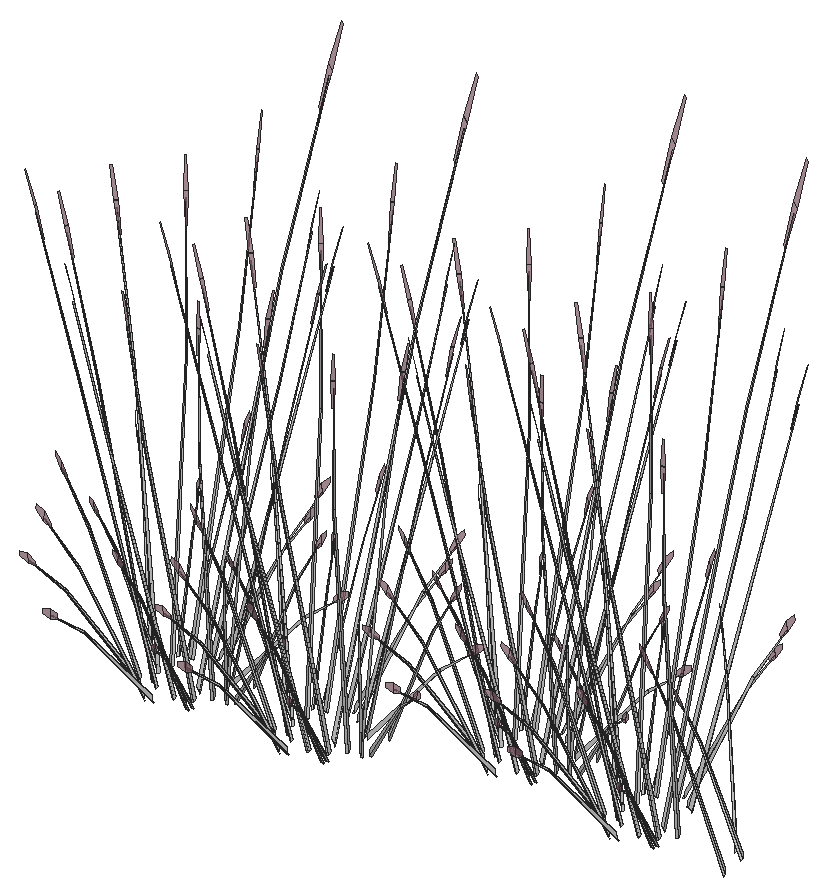
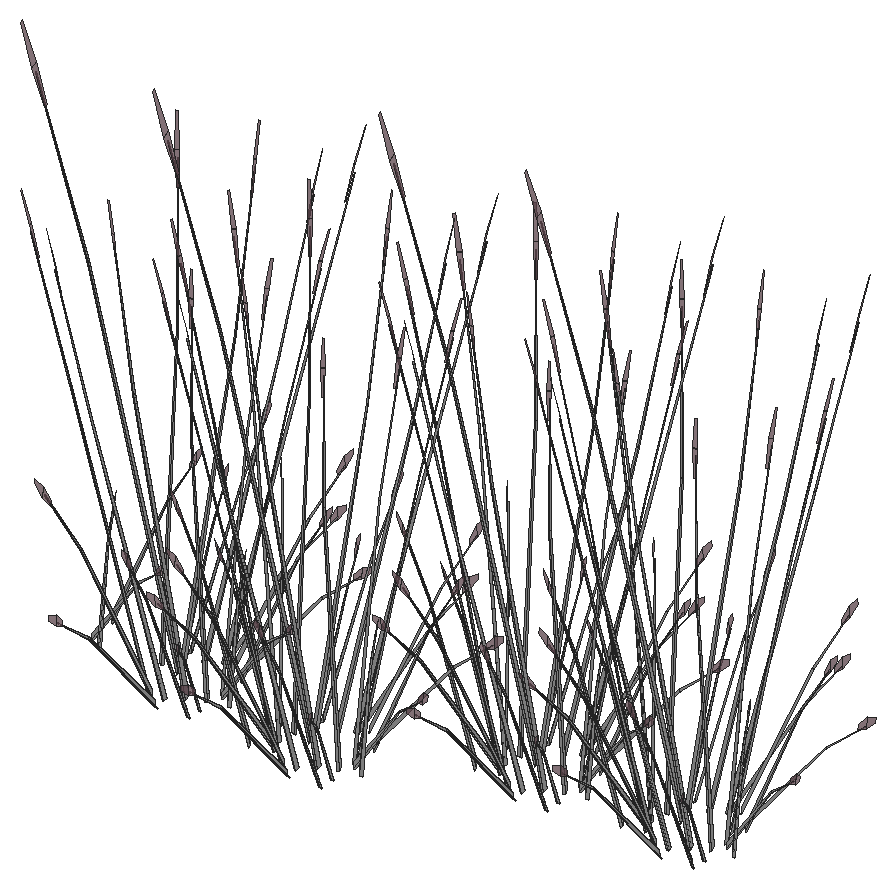
# SketchUp Ruby script. Lengths in inches.
U = 1.inch
M = Sketchup.active_model
def pt(a) = Geom::Point3d.new(a.map { |v| v * U })
def face(e, loops, mat)
  f = e.add_face(loops[0].map { |a| pt(a) })
  loops[1..].each { |l| e.add_face(l.map { |a| pt(a) }).erase! }
  f.material = f.back_material = mat if mat
  f
end
# faces: each face lists its corners as indices into pts; further lists are holes
def faces(e, pts, list, mat = nil) = list.each { |f| face(e, (f[0].is_a?(Array) ? f : [f]).map { |l| l.map { |i| pts[i] } }, mat) }
# xy, xz, yz: faces in a plane at the given z, y or x. An outline is a flat list of corners, or four numbers for a rectangle; further outlines are holes
def ring(l) = l.size == 4 ? [[l[0], l[1]], [l[2], l[1]], [l[2], l[3]], [l[0], l[3]]] : l.each_slice(2).to_a
def flat(e, list, mat, &to3) = list.each { |f| face(e, (f[0].is_a?(Array) ? f : [f]).map { |l| ring(l).map { |u, v| to3.(u, v) } }, mat) }
def xy(e, z, list, mat = nil) = flat(e, list, mat) { |x, y| [x, y, z] }
def xz(e, y, list, mat = nil) = flat(e, list, mat) { |x, z| [x, y, z] }
def yz(e, x, list, mat = nil) = flat(e, list, mat) { |y, z| [x, y, z] }
def lines(e, pts, list) = list.each { |a, b| e.add_line(pt(pts[a]), pt(pts[b])) }
# prism: a flat outline (further loops are holes) pulled along v
def prism(e, loops, v, mat = nil)
  f = face(e, loops, mat); d = Geom::Vector3d.new(v.map { |x| x * U })
  f.pushpull(f.normal.samedirection?(d) ? d.length : -d.length)
end
def box(e, o, s, mat = nil) = prism(e, [[o, [o[0] + s[0], o[1], o[2]], [o[0] + s[0], o[1] + s[1], o[2]], [o[0], o[1] + s[1], o[2]]]], [0, 0, s[2]], mat)
def at(x, y, z, deg = 0) = Geom::Transformation.translation(pt([x, y, z])) * Geom::Transformation.rotation(ORIGIN, Z_AXIS, deg.degrees)
def axes(o, x, y, z) = Geom::Transformation.new([*x, 0, *y, 0, *z, 0, *pt(o).to_a, 1])
def part(name) = M.definitions.add(name)
# library, detail: a bought-in or finely detailed component or shape, given as its bounding box
def library(name, o, s) = part(name).tap { |d| box(d.entities, o, s) }
def detail(e, o, s) = box(e.add_group.entities, o, s)
def put(e, d, t, mat = nil) = e.add_instance(d, t).tap { |i| i.material = mat if mat }
def group(e, t, mat = nil) = e.add_group.tap { |g| g.transformation = t; g.material = mat if mat }.entities
root = M.entities
M.materials.add("LightPink_Translucent").color = [144, 107, 117]
M.materials["LightPink_Translucent"].alpha = 0.75
M.materials.add("[_0053_Ivory_]").color = [200, 200, 200]
c1 = part("blade")
p = [[2.15,0.21,22],[0,0.17,0],[0.09,0.45,0],[2.18,0.31,22],[2.29,0.31,22],[0.38,0.45,0],
  [2.48,0.24,33],[2.49,0.24,33],[2.48,0.22,33]]
faces(c1.entities,p,[[0,1,2,3],[4,5,2,3],[6,3,4,7],[8,0,3,6]])
c2 = part("seeds")
p = [[0.3,-0.1,1.38],[-0.01,-0.03,1.59],[-0.01,-0.03,0.03],[0.14,-0.07,-0.07],[0.29,-0.03,3],[0.15,0.01,3.11]]
faces(c2.entities,p,[[0,1,2,3],[1,0,4,5]],"LightPink_Translucent")
c3 = part("blade with seeds")
put(c3.entities,c1,at(0,0,0))
put(c3.entities,c2,axes([2.4,0.25,30.99],[1.5799,-0.05474,1.17369],[-0.12525,1.92788,0.29478],[-0.07173,-0.02425,1.56792]))
put(root,c3,axes([417.2,98.36,131.37],[-0.09918,0.08165,1.74944],[0.00844,0.59653,-0.27667],[-0.22734,0.07758,0.14031]),"[_0053_Ivory_]")
put(root,c3,axes([416.1,98.96,131.36],[0.07751,0.01687,1.77383],[0.23978,0.55562,-0.16761],[-0.15867,0.14583,0.31391]),"[_0053_Ivory_]")
put(root,c3,axes([417.67,95.875,131.36],[0.04503,0.06276,1.77383],[-0.21706,0.56413,-0.16761],[-0.21983,0.00408,0.31391]),"[_0053_Ivory_]")
put(root,c3,axes([418.17,95.5,131.37],[-0.13068,-0.00444,1.74944],[-0.41604,0.44388,-0.27667],[-0.22198,-0.0907,0.14031]),"[_0053_Ivory_]")
put(root,c3,axes([417.84,97.79,131.6875],[0.30559,0.56943,-0.1216],[-0.54237,0.27983,-0.67495],[-0.22856,0.07513,1.02557]),"[_0053_Ivory_]")
put(root,c3,axes([418.52,96.61,131.6875],[-0.03252,0.63953,-0.1216],[-0.61574,-0.01748,-0.67495],[-0.23714,-0.04442,1.02557]),"[_0053_Ivory_]")
put(root,c3,axes([417.22,100.58,131.37],[-0.0151,0.12444,1.74944],[0.42844,0.43292,-0.27667],[-0.11216,0.20472,0.14031]),"[_0053_Ivory_]")
put(root,c3,axes([419.73,95.67,132.08],[-0.40534,0.60286,-0.13619],[-0.58702,-0.34732,-0.75594],[-0.20405,-0.17032,1.14864]),"[_0053_Ivory_]")
put(root,c3,axes([417.86,99.14,131.6875],[0.56181,0.34675,-0.1216],[-0.32367,0.50216,-0.67495],[-0.15873,0.17455,1.02557]),"[_0053_Ivory_]")
put(root,c3,axes([419.57,94.24,131.36],[-0.01133,0.07538,1.77383],[-0.55883,0.27355,-0.16761],[-0.16445,-0.13983,0.31391]),"[_0053_Ivory_]")
put(root,c3,axes([417.17,101.86,131.36],[0.0689,-0.03797,1.77383],[0.5695,0.25254,-0.16761],[-0.01338,0.21027,0.31391]),"[_0053_Ivory_]")
put(root,c3,axes([420.21,94.53,131.37],[-0.0929,-0.08817,1.74944],[-0.61994,0.0559,-0.27667],[-0.09894,-0.21089,0.14031]),"[_0053_Ivory_]")
put(root,c3,axes([418.59,100.3,132.05],[0.6675,0.03116,-0.13498],[-0.01824,0.58993,-0.74919],[-0.04637,0.2272,1.13838]),"[_0053_Ivory_]")
put(root,c3,axes([421.15,95.89,131.6875],[-0.59433,0.29278,-0.1216],[-0.29207,-0.51964,-0.67495],[-0.07842,-0.21898,1.02557]),"[_0053_Ivory_]")
put(root,c3,axes([419.68,102.125,131.37],[0.07699,0.10127,1.74944],[0.6213,0.03978,-0.27667],[0.06248,0.22333,0.14031]),"[_0053_Ivory_]")
put(root,c3,axes([419.82,100.96,131.6875],[0.59433,-0.29278,-0.1216],[0.29207,0.51964,-0.67495],[0.07842,0.21898,1.02557]),"[_0053_Ivory_]")
put(root,c3,axes([422.86,95.16,131.36],[-0.06168,0.04803,1.77383],[-0.60432,-0.16205,-0.16761],[-0.02188,-0.20961,0.31391]),"[_0053_Ivory_]")
put(root,c3,axes([422.38,96.55,131.6875],[-0.6675,-0.03116,-0.1216],[0.01824,-0.58993,-0.67495],[0.04637,-0.2272,1.02557]),"[_0053_Ivory_]")
put(root,c3,axes([421.64,97.76,131.13],[-0.52482,-0.32674,1.38283],[0.55416,-0.50872,0.59665],[0.16933,0.30658,1.33663]),"[_0053_Ivory_]")
put(root,c3,axes([420.76,101.39,131.36],[0.0018,-0.07613,1.77383],[0.52048,-0.3359,-0.16761],[0.18079,0.11989,0.31391]),"[_0053_Ivory_]")
put(root,c3,axes([422.99,95.61,131.37],[-0.00586,-0.12516,1.74944],[-0.49517,-0.36172,-0.27667],[0.07656,-0.21927,0.14031]),"[_0053_Ivory_]")
put(root,c3,axes([429.41,98.36,131.37],[-0.09918,0.08165,1.74944],[0.00844,0.59653,-0.27667],[-0.22734,0.07758,0.14031]),"[_0053_Ivory_]")
put(root,c3,axes([421.23,100.9375,131.6875],[0.36191,-0.53827,-0.1216],[0.52412,0.3101,-0.67495],[0.18219,0.15207,1.02557]),"[_0053_Ivory_]")
put(root,c3,axes([423.11,97.71,131.6875],[-0.56181,-0.34675,-0.1216],[0.32367,-0.50216,-0.67495],[0.15873,-0.17455,1.02557]),"[_0053_Ivory_]")
put(root,c3,axes([428.3125,98.96,131.36],[0.07751,0.01687,1.77383],[0.23978,0.55562,-0.16761],[-0.15867,0.14583,0.31391]),"[_0053_Ivory_]")
put(root,c3,axes([429.88,95.875,131.36],[0.04503,0.06276,1.77383],[-0.21706,0.56413,-0.16761],[-0.21983,0.00408,0.31391]),"[_0053_Ivory_]")
put(root,c3,axes([430.39,95.5,131.37],[-0.13068,-0.00444,1.74944],[-0.41604,0.44388,-0.27667],[-0.22198,-0.0907,0.14031]),"[_0053_Ivory_]")
put(root,c3,axes([430.05,97.79,131.6875],[0.30559,0.56943,-0.1216],[-0.54237,0.27983,-0.67495],[-0.22856,0.07513,1.02557]),"[_0053_Ivory_]")
put(root,c3,axes([430.74,96.61,131.6875],[-0.03252,0.63953,-0.1216],[-0.61574,-0.01748,-0.67495],[-0.23714,-0.04442,1.02557]),"[_0053_Ivory_]")
put(root,c3,axes([424.49,97.56,131.36],[-0.07933,-0.00478,1.77383],[-0.32942,-0.51175,-0.16761],[0.13229,-0.16826,0.31391]),"[_0053_Ivory_]")
put(root,c3,axes([422.45,100.24,131.6875],[0.03252,-0.63953,-0.1216],[0.61574,0.01748,-0.67495],[0.23714,0.04442,1.02557]),"[_0053_Ivory_]")
put(root,c3,axes([423.13,99.0625,131.6875],[-0.30559,-0.56943,-0.1216],[0.54237,-0.27983,-0.67495],[0.22856,-0.07513,1.02557]),"[_0053_Ivory_]")
put(root,c3,axes([422.98,99.86,131.37],[0.13029,-0.01064,1.74944],[0.35737,-0.48855,-0.27667],[0.23175,0.06449,0.14031]),"[_0053_Ivory_]")
put(root,c3,axes([429.43,100.58,131.37],[-0.0151,0.12444,1.74944],[0.42844,0.43292,-0.27667],[-0.11216,0.20472,0.14031]),"[_0053_Ivory_]")
put(root,c3,axes([431.94,95.67,132.08],[-0.40534,0.60286,-0.13619],[-0.58702,-0.34732,-0.75594],[-0.20405,-0.17032,1.14864]),"[_0053_Ivory_]")
put(root,c3,axes([430.07,99.14,131.6875],[0.56181,0.34675,-0.1216],[-0.32367,0.50216,-0.67495],[-0.15873,0.17455,1.02557]),"[_0053_Ivory_]")
put(root,c3,axes([424.35,100.75,131.36],[-0.05492,-0.05505,1.77383],[0.12013,-0.59013,-0.16761],[0.21632,-0.0377,0.31391]),"[_0053_Ivory_]")
put(root,c3,axes([431.78,94.24,131.36],[-0.01133,0.07538,1.77383],[-0.55883,0.27355,-0.16761],[-0.16445,-0.13983,0.31391]),"[_0053_Ivory_]")
put(root,c3,axes([424.79,98.17,131.37],[0.08428,-0.09579,1.74944],[-0.10787,-0.58756,-0.27667],[0.21147,-0.1114,0.14031]),"[_0053_Ivory_]")
put(root,c3,axes([429.38,101.86,131.36],[0.0689,-0.03797,1.77383],[0.5695,0.25254,-0.16761],[-0.01338,0.21027,0.31391]),"[_0053_Ivory_]")
put(root,c3,axes([432.42,94.53,131.37],[-0.0929,-0.08817,1.74944],[-0.61994,0.0559,-0.27667],[-0.09894,-0.21089,0.14031]),"[_0053_Ivory_]")
put(root,c3,axes([430.8,100.3,132.05],[0.6675,0.03116,-0.13498],[-0.01824,0.58993,-0.74919],[-0.04637,0.2272,1.13838]),"[_0053_Ivory_]")
put(root,c3,axes([433.36,95.89,131.6875],[-0.59433,0.29278,-0.1216],[-0.29207,-0.51964,-0.67495],[-0.07842,-0.21898,1.02557]),"[_0053_Ivory_]")
put(root,c3,axes([431.9,102.125,131.37],[0.07699,0.10127,1.74944],[0.6213,0.03978,-0.27667],[0.06248,0.22333,0.14031]),"[_0053_Ivory_]")
put(root,c3,axes([432.04,100.96,131.6875],[0.59433,-0.29278,-0.1216],[0.29207,0.51964,-0.67495],[0.07842,0.21898,1.02557]),"[_0053_Ivory_]")
put(root,c3,axes([435.07,95.16,131.36],[-0.06168,0.04803,1.77383],[-0.60432,-0.16205,-0.16761],[-0.02188,-0.20961,0.31391]),"[_0053_Ivory_]")
put(root,c3,axes([434.6,96.55,131.6875],[-0.6675,-0.03116,-0.1216],[0.01824,-0.58993,-0.67495],[0.04637,-0.2272,1.02557]),"[_0053_Ivory_]")
put(root,c3,axes([433.86,97.76,131.13],[-0.52482,-0.32674,1.38283],[0.55416,-0.50872,0.59665],[0.16933,0.30658,1.33663]),"[_0053_Ivory_]")
put(root,c3,axes([432.97,101.39,131.36],[0.0018,-0.07613,1.77383],[0.52048,-0.3359,-0.16761],[0.18079,0.11989,0.31391]),"[_0053_Ivory_]")
put(root,c3,axes([435.2,95.61,131.37],[-0.00586,-0.12516,1.74944],[-0.49517,-0.36172,-0.27667],[0.07656,-0.21927,0.14031]),"[_0053_Ivory_]")
put(root,c3,axes([433.45,100.9375,131.6875],[0.36191,-0.53827,-0.1216],[0.52412,0.3101,-0.67495],[0.18219,0.15207,1.02557]),"[_0053_Ivory_]")
put(root,c3,axes([435.32,97.71,131.6875],[-0.56181,-0.34675,-0.1216],[0.32367,-0.50216,-0.67495],[0.15873,-0.17455,1.02557]),"[_0053_Ivory_]")
put(root,c3,axes([442.82,105.17,131.37],[-0.09918,0.08165,1.74944],[0.00844,0.59653,-0.27667],[-0.22734,0.07758,0.14031]),"[_0053_Ivory_]")
put(root,c3,axes([436.71,97.56,131.36],[-0.07933,-0.00478,1.77383],[-0.32942,-0.51175,-0.16761],[0.13229,-0.16826,0.31391]),"[_0053_Ivory_]")
put(root,c3,axes([441.72,105.77,131.36],[0.07751,0.01687,1.77383],[0.23978,0.55562,-0.16761],[-0.15867,0.14583,0.31391]),"[_0053_Ivory_]")
put(root,c3,axes([434.66,100.24,131.6875],[0.03252,-0.63953,-0.1216],[0.61574,0.01748,-0.67495],[0.23714,0.04442,1.02557]),"[_0053_Ivory_]")
put(root,c3,axes([435.35,99.0625,131.6875],[-0.30559,-0.56943,-0.1216],[0.54237,-0.27983,-0.67495],[0.22856,-0.07513,1.02557]),"[_0053_Ivory_]")
put(root,c3,axes([443.29,102.68,131.36],[0.04503,0.06276,1.77383],[-0.21706,0.56413,-0.16761],[-0.21983,0.00408,0.31391]),"[_0053_Ivory_]")
put(root,c3,axes([443.79,102.31,131.37],[-0.13068,-0.00444,1.74944],[-0.41604,0.44388,-0.27667],[-0.22198,-0.0907,0.14031]),"[_0053_Ivory_]")
put(root,c3,axes([443.45,104.6,131.6875],[0.30559,0.56943,-0.1216],[-0.54237,0.27983,-0.67495],[-0.22856,0.07513,1.02557]),"[_0053_Ivory_]")
put(root,c3,axes([435.2,99.86,131.37],[0.13029,-0.01064,1.74944],[0.35737,-0.48855,-0.27667],[0.23175,0.06449,0.14031]),"[_0053_Ivory_]")
put(root,c3,axes([444.14,103.42,131.6875],[-0.03252,0.63953,-0.1216],[-0.61574,-0.01748,-0.67495],[-0.23714,-0.04442,1.02557]),"[_0053_Ivory_]")
put(root,c3,axes([436.5625,100.75,131.36],[-0.05492,-0.05505,1.77383],[0.12013,-0.59013,-0.16761],[0.21632,-0.0377,0.31391]),"[_0053_Ivory_]")
put(root,c3,axes([442.83,107.39,131.37],[-0.0151,0.12444,1.74944],[0.42844,0.43292,-0.27667],[-0.11216,0.20472,0.14031]),"[_0053_Ivory_]")
put(root,c3,axes([437.01,98.17,131.37],[0.08428,-0.09579,1.74944],[-0.10787,-0.58756,-0.27667],[0.21147,-0.1114,0.14031]),"[_0053_Ivory_]")
put(root,c3,axes([445.34,102.48,132.08],[-0.40534,0.60286,-0.13619],[-0.58702,-0.34732,-0.75594],[-0.20405,-0.17032,1.14864]),"[_0053_Ivory_]")
put(root,c3,axes([443.48,105.95,131.6875],[0.56181,0.34675,-0.1216],[-0.32367,0.50216,-0.67495],[-0.15873,0.17455,1.02557]),"[_0053_Ivory_]")
put(root,c3,axes([445.1875,101.05,131.36],[-0.01133,0.07538,1.77383],[-0.55883,0.27355,-0.16761],[-0.16445,-0.13983,0.31391]),"[_0053_Ivory_]")
put(root,c3,axes([442.79,108.67,131.36],[0.0689,-0.03797,1.77383],[0.5695,0.25254,-0.16761],[-0.01338,0.21027,0.31391]),"[_0053_Ivory_]")
put(root,c3,axes([445.82,101.34,131.37],[-0.0929,-0.08817,1.74944],[-0.61994,0.0559,-0.27667],[-0.09894,-0.21089,0.14031]),"[_0053_Ivory_]")
put(root,c3,axes([444.2,107.11,132.05],[0.6675,0.03116,-0.13498],[-0.01824,0.58993,-0.74919],[-0.04637,0.2272,1.13838]),"[_0053_Ivory_]")
put(root,c3,axes([446.77,102.7,131.6875],[-0.59433,0.29278,-0.1216],[-0.29207,-0.51964,-0.67495],[-0.07842,-0.21898,1.02557]),"[_0053_Ivory_]")
put(root,c3,axes([445.3,108.93,131.37],[0.07699,0.10127,1.74944],[0.6213,0.03978,-0.27667],[0.06248,0.22333,0.14031]),"[_0053_Ivory_]")
put(root,c3,axes([445.4375,107.77,131.6875],[0.59433,-0.29278,-0.1216],[0.29207,0.51964,-0.67495],[0.07842,0.21898,1.02557]),"[_0053_Ivory_]")
put(root,c3,axes([448.48,101.97,131.36],[-0.06168,0.04803,1.77383],[-0.60432,-0.16205,-0.16761],[-0.02188,-0.20961,0.31391]),"[_0053_Ivory_]")
put(root,c3,axes([448,103.36,131.6875],[-0.6675,-0.03116,-0.1216],[0.01824,-0.58993,-0.67495],[0.04637,-0.2272,1.02557]),"[_0053_Ivory_]")
put(root,c3,axes([447.26,104.57,131.13],[-0.52482,-0.32674,1.38283],[0.55416,-0.50872,0.59665],[0.16933,0.30658,1.33663]),"[_0053_Ivory_]")
put(root,c3,axes([446.38,108.2,131.36],[0.0018,-0.07613,1.77383],[0.52048,-0.3359,-0.16761],[0.18079,0.11989,0.31391]),"[_0053_Ivory_]")
put(root,c3,axes([448.61,102.42,131.37],[-0.00586,-0.12516,1.74944],[-0.49517,-0.36172,-0.27667],[0.07656,-0.21927,0.14031]),"[_0053_Ivory_]")
put(root,c3,axes([446.85,107.75,131.6875],[0.36191,-0.53827,-0.1216],[0.52412,0.3101,-0.67495],[0.18219,0.15207,1.02557]),"[_0053_Ivory_]")
put(root,c3,axes([448.73,104.52,131.6875],[-0.56181,-0.34675,-0.1216],[0.32367,-0.50216,-0.67495],[0.15873,-0.17455,1.02557]),"[_0053_Ivory_]")
put(root,c3,axes([455.3,103.35,131.37],[-0.09918,0.08165,1.74944],[0.00844,0.59653,-0.27667],[-0.22734,0.07758,0.14031]),"[_0053_Ivory_]")
put(root,c3,axes([454.2,103.95,131.36],[0.07751,0.01687,1.77383],[0.23978,0.55562,-0.16761],[-0.15867,0.14583,0.31391]),"[_0053_Ivory_]")
put(root,c3,axes([455.77,100.87,131.36],[0.04503,0.06276,1.77383],[-0.21706,0.56413,-0.16761],[-0.21983,0.00408,0.31391]),"[_0053_Ivory_]")
put(root,c3,axes([456.27,100.49,131.37],[-0.13068,-0.00444,1.74944],[-0.41604,0.44388,-0.27667],[-0.22198,-0.0907,0.14031]),"[_0053_Ivory_]")
put(root,c3,axes([455.9375,102.78,131.6875],[0.30559,0.56943,-0.1216],[-0.54237,0.27983,-0.67495],[-0.22856,0.07513,1.02557]),"[_0053_Ivory_]")
put(root,c3,axes([456.625,101.6,131.6875],[-0.03252,0.63953,-0.1216],[-0.61574,-0.01748,-0.67495],[-0.23714,-0.04442,1.02557]),"[_0053_Ivory_]")
put(root,c3,axes([450.11,104.37,131.36],[-0.07933,-0.00478,1.77383],[-0.32942,-0.51175,-0.16761],[0.13229,-0.16826,0.31391]),"[_0053_Ivory_]")
put(root,c3,axes([448.0625,107.05,131.6875],[0.03252,-0.63953,-0.1216],[0.61574,0.01748,-0.67495],[0.23714,0.04442,1.02557]),"[_0053_Ivory_]")
put(root,c3,axes([448.75,105.87,131.6875],[-0.30559,-0.56943,-0.1216],[0.54237,-0.27983,-0.67495],[0.22856,-0.07513,1.02557]),"[_0053_Ivory_]")
put(root,c3,axes([448.6,106.67,131.37],[0.13029,-0.01064,1.74944],[0.35737,-0.48855,-0.27667],[0.23175,0.06449,0.14031]),"[_0053_Ivory_]")
put(root,c3,axes([455.32,105.58,131.37],[-0.0151,0.12444,1.74944],[0.42844,0.43292,-0.27667],[-0.11216,0.20472,0.14031]),"[_0053_Ivory_]")
put(root,c3,axes([457.83,100.66,132.08],[-0.40534,0.60286,-0.13619],[-0.58702,-0.34732,-0.75594],[-0.20405,-0.17032,1.14864]),"[_0053_Ivory_]")
put(root,c3,axes([449.97,107.5625,131.36],[-0.05492,-0.05505,1.77383],[0.12013,-0.59013,-0.16761],[0.21632,-0.0377,0.31391]),"[_0053_Ivory_]")
put(root,c3,axes([455.96,104.13,131.6875],[0.56181,0.34675,-0.1216],[-0.32367,0.50216,-0.67495],[-0.15873,0.17455,1.02557]),"[_0053_Ivory_]")
put(root,c3,axes([450.41,104.98,131.37],[0.08428,-0.09579,1.74944],[-0.10787,-0.58756,-0.27667],[0.21147,-0.1114,0.14031]),"[_0053_Ivory_]")
put(root,c3,axes([457.67,99.23,131.36],[-0.01133,0.07538,1.77383],[-0.55883,0.27355,-0.16761],[-0.16445,-0.13983,0.31391]),"[_0053_Ivory_]")
put(root,c3,axes([455.27,106.85,131.36],[0.0689,-0.03797,1.77383],[0.5695,0.25254,-0.16761],[-0.01338,0.21027,0.31391]),"[_0053_Ivory_]")
put(root,c3,axes([458.3,99.52,131.37],[-0.0929,-0.08817,1.74944],[-0.61994,0.0559,-0.27667],[-0.09894,-0.21089,0.14031]),"[_0053_Ivory_]")
put(root,c3,axes([456.6875,105.29,132.05],[0.6675,0.03116,-0.13498],[-0.01824,0.58993,-0.74919],[-0.04637,0.2272,1.13838]),"[_0053_Ivory_]")
put(root,c3,axes([459.25,100.88,131.6875],[-0.59433,0.29278,-0.1216],[-0.29207,-0.51964,-0.67495],[-0.07842,-0.21898,1.02557]),"[_0053_Ivory_]")
put(root,c3,axes([457.78,107.11,131.37],[0.07699,0.10127,1.74944],[0.6213,0.03978,-0.27667],[0.06248,0.22333,0.14031]),"[_0053_Ivory_]")
put(root,c3,axes([457.92,105.95,131.6875],[0.59433,-0.29278,-0.1216],[0.29207,0.51964,-0.67495],[0.07842,0.21898,1.02557]),"[_0053_Ivory_]")
put(root,c3,axes([460.96,100.15,131.36],[-0.06168,0.04803,1.77383],[-0.60432,-0.16205,-0.16761],[-0.02188,-0.20961,0.31391]),"[_0053_Ivory_]")
put(root,c3,axes([460.48,101.54,131.6875],[-0.6675,-0.03116,-0.1216],[0.01824,-0.58993,-0.67495],[0.04637,-0.2272,1.02557]),"[_0053_Ivory_]")
put(root,c3,axes([459.74,102.75,131.13],[-0.52482,-0.32674,1.38283],[0.55416,-0.50872,0.59665],[0.16933,0.30658,1.33663]),"[_0053_Ivory_]")
put(root,c3,axes([458.86,106.38,131.36],[0.0018,-0.07613,1.77383],[0.52048,-0.3359,-0.16761],[0.18079,0.11989,0.31391]),"[_0053_Ivory_]")
put(root,c3,axes([461.09,100.6,131.37],[-0.00586,-0.12516,1.74944],[-0.49517,-0.36172,-0.27667],[0.07656,-0.21927,0.14031]),"[_0053_Ivory_]")
put(root,c3,axes([466.8125,102.49,131.37],[-0.09918,0.08165,1.74944],[0.00844,0.59653,-0.27667],[-0.22734,0.07758,0.14031]),"[_0053_Ivory_]")
put(root,c3,axes([465.71,103.09,131.36],[0.07751,0.01687,1.77383],[0.23978,0.55562,-0.16761],[-0.15867,0.14583,0.31391]),"[_0053_Ivory_]")
put(root,c3,axes([459.33,105.93,131.6875],[0.36191,-0.53827,-0.1216],[0.52412,0.3101,-0.67495],[0.18219,0.15207,1.02557]),"[_0053_Ivory_]")
put(root,c3,axes([467.28,100.01,131.36],[0.04503,0.06276,1.77383],[-0.21706,0.56413,-0.16761],[-0.21983,0.00408,0.31391]),"[_0053_Ivory_]")
put(root,c3,axes([461.21,102.7,131.6875],[-0.56181,-0.34675,-0.1216],[0.32367,-0.50216,-0.67495],[0.15873,-0.17455,1.02557]),"[_0053_Ivory_]")
